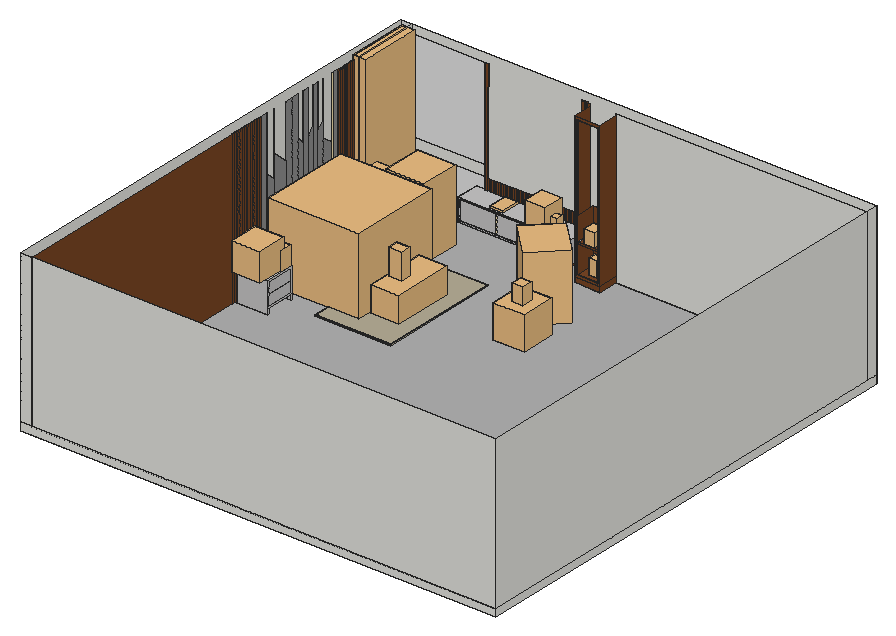
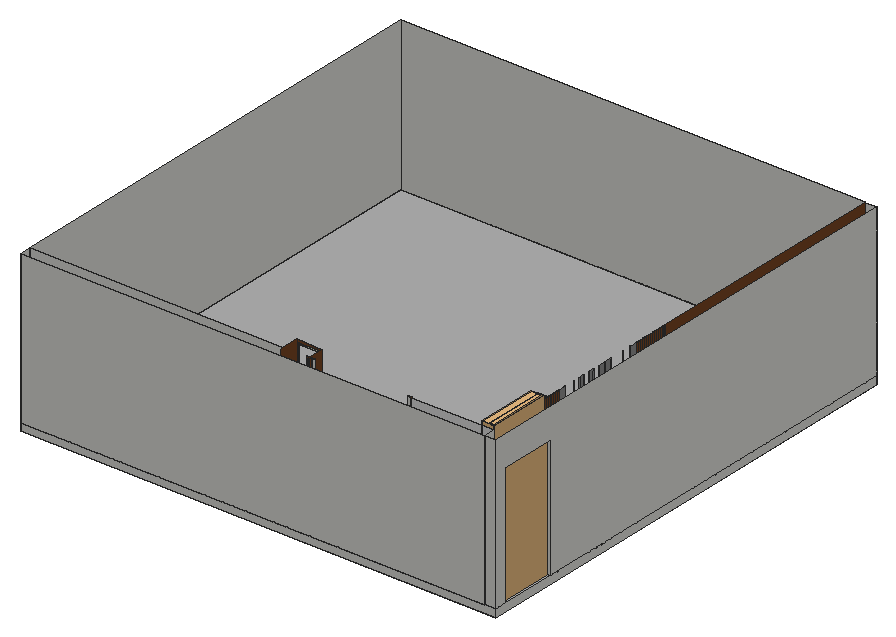
# SketchUp Ruby script. Lengths in inches.
U = 1.inch
M = Sketchup.active_model
def pt(a) = Geom::Point3d.new(a.map { |v| v * U })
def face(e, loops, mat)
  f = e.add_face(loops[0].map { |a| pt(a) })
  loops[1..].each { |l| e.add_face(l.map { |a| pt(a) }).erase! }
  f.material = f.back_material = mat if mat
  f
end
# faces: each face lists its corners as indices into pts; further lists are holes
def faces(e, pts, list, mat = nil) = list.each { |f| face(e, (f[0].is_a?(Array) ? f : [f]).map { |l| l.map { |i| pts[i] } }, mat) }
# xy, xz, yz: faces in a plane at the given z, y or x. An outline is a flat list of corners, or four numbers for a rectangle; further outlines are holes
def ring(l) = l.size == 4 ? [[l[0], l[1]], [l[2], l[1]], [l[2], l[3]], [l[0], l[3]]] : l.each_slice(2).to_a
def flat(e, list, mat, &to3) = list.each { |f| face(e, (f[0].is_a?(Array) ? f : [f]).map { |l| ring(l).map { |u, v| to3.(u, v) } }, mat) }
def xy(e, z, list, mat = nil) = flat(e, list, mat) { |x, y| [x, y, z] }
def xz(e, y, list, mat = nil) = flat(e, list, mat) { |x, z| [x, y, z] }
def yz(e, x, list, mat = nil) = flat(e, list, mat) { |y, z| [x, y, z] }
def lines(e, pts, list) = list.each { |a, b| e.add_line(pt(pts[a]), pt(pts[b])) }
# prism: a flat outline (further loops are holes) pulled along v
def prism(e, loops, v, mat = nil)
  f = face(e, loops, mat); d = Geom::Vector3d.new(v.map { |x| x * U })
  f.pushpull(f.normal.samedirection?(d) ? d.length : -d.length)
end
def box(e, o, s, mat = nil) = prism(e, [[o, [o[0] + s[0], o[1], o[2]], [o[0] + s[0], o[1] + s[1], o[2]], [o[0], o[1] + s[1], o[2]]]], [0, 0, s[2]], mat)
def at(x, y, z, deg = 0) = Geom::Transformation.translation(pt([x, y, z])) * Geom::Transformation.rotation(ORIGIN, Z_AXIS, deg.degrees)
def axes(o, x, y, z) = Geom::Transformation.new([*x, 0, *y, 0, *z, 0, *pt(o).to_a, 1])
def part(name) = M.definitions.add(name)
# library, detail: a bought-in or finely detailed component or shape, given as its bounding box
def library(name, o, s) = part(name).tap { |d| box(d.entities, o, s) }
def detail(e, o, s) = box(e.add_group.entities, o, s)
def put(e, d, t, mat = nil) = e.add_instance(d, t).tap { |i| i.material = mat if mat }
def group(e, t, mat = nil) = e.add_group.tap { |g| g.transformation = t; g.material = mat if mat }.entities
root = M.entities
M.materials.add("Ashlee 5_ x 8_").color = [182, 173, 150]
M.materials.add("Emissive").color = [234, 236, 196]
M.materials.add("Generic").color = [198, 197, 197]
M.materials.add("Gold 10k").color = [251, 232, 180]
M.materials.add("Tiles Simple J01 100cm").color = [178, 178, 178]
M.materials.add("[Color M01]").color = [226, 226, 226]
M.materials.add("[Color M04]").color = [142, 142, 142]
M.materials.add("[Wood Veneer 01]").color = [120, 70, 37]
c1 = library("Window 46-12",[-37.28,-2.15,0],[74.56,4.3,92.91])
c2 = library("Granville Side Chair",[-10.69,-11.14,0],[21.38,22.37,32.46])
c3 = part(" rug 5'x8'\#1")
xy(c3.entities,0,[[0,0,60,96]],"Ashlee 5_ x 8_")
xy(c3.entities,0.75,[[0.25,0.25,59.75,95.75]],"Ashlee 5_ x 8_")
xz(c3.entities,0,[[0,0,60,0.5]],"Ashlee 5_ x 8_")
xz(c3.entities,96,[[0,0,60,0.5]],"Ashlee 5_ x 8_")
yz(c3.entities,0,[[0,0,96,0.5]],"Ashlee 5_ x 8_")
yz(c3.entities,60,[[0,0,96,0.5]],"Ashlee 5_ x 8_")
p = [[59.99,0.01,0.56],[0.01,0.01,0.56],[0,0,0.5],[60,0,0.5],[0.01,95.99,0.56],[0,96,0.5],
  [59.99,95.99,0.56],[60,96,0.5],[0.03,0.03,0.625],[0.03,95.97,0.625],[59.97,0.03,0.625],[59.93,0.07,0.68],
  [0.07,0.07,0.68],[0.07,95.93,0.68],[59.93,95.93,0.68],[59.97,95.97,0.625],[0.125,0.125,0.72],[0.125,95.875,0.72],
  [59.81,0.19,0.74],[0.19,0.19,0.74],[59.875,0.125,0.72],[0.19,95.81,0.74],[59.81,95.81,0.74],[59.875,95.875,0.72],
  [0.25,0.25,0.75],[0.25,95.75,0.75],[59.75,0.25,0.75],[59.75,95.75,0.75]]
faces(c3.entities,p,[[0,1,2,3],[1,4,5,2],[6,0,3,7],[4,6,7,5],[8,9,4,1],[10,8,1,0],[11,12,8,10],[12,13,9,8],
  [14,11,10,15],[15,10,0,6],[13,14,15,9],[9,15,6,4],[16,17,13,12],[18,19,16,20],[20,16,12,11],[19,21,17,16],
  [22,18,20,23],[23,20,11,14],[24,25,21,19],[26,24,19,18],[27,26,18,22],[21,22,23,17],[25,27,22,21],[17,23,14,13]],"Ashlee 5_ x 8_")
c4 = library("Granville Bridge Armchair",[-12.42,-11.18,0],[24.84,22.36,32.46])
c5 = library("Bed 003",[-38.05,-87.1,0],[75.86,87.1,55.12])
c6 = library("Negro Coffee Table",[-11.41,-11.39,0.01],[22.79,22.78,16.72])
c7 = library("Eva Bench",[-23.95,-11.14,0],[47.9,22.28,20.23])
c8 = library("Curtains 005",[-39.6,-1.86,0],[79.2,3.72,117.07])
c9 = library("Curtains 47-24",[-33.71,-5.15,0],[67.39,10.25,93.3])
c10 = library("Milk Jug 92-23",[-3.1,-3.1,0],[6.18,6.2,11.88])
c11 = library("Vase 20-10",[-4.83,-4.83,0],[9.66,9.66,14.63])
c12 = library("Vase Roses 63-11",[-11.16,-11.66,0.01],[22.4,23.28,22.51])
c13 = library("Vase 003",[-5.32,-3.71,0],[10.44,8.14,20.48])
c14 = library("Calla Lilies 63-10",[-4.34,-4.49,0],[8.67,8.83,13.09])
c15 = library("Vase 005",[-3.71,-4.3,0.02],[8.35,9.45,10.71])
c16 = library("Book 298 011 003",[-5.11,-7.51,-0.03],[10.21,15.02,1.37])
c17 = library("Vase 012",[-2.85,-2.85,0],[5.7,5.7,9.98])
c18 = library("Vase Calla Lilies 21-24",[-7.55,-8.25,0],[16.06,16.68,17.86])
xy(root,-6,[[0,0,376.875,376.875]])
xy(root,0,[[0,0,0,322.76,9,322.76,9,321.04,8.75,321.04,8.75,318.98,9,318.98,9,317.73,8.75,317.73,8.75,316.79,9,316.79,9,315.55,8.75,315.55,8.75,314.73,9,314.73,9,313.48,8.75,313.48,8.75,312.66,9,312.66,9,311.42,9.0625,311.42,9.0625,310.66,9,310.66,9,309.42,9.0625,309.42,9.0625,308.48,9,308.48,9,307.23,9.0625,307.23,9.0625,306.48,9,306.48,9,305.23,9.0625,305.23,9.0625,304.35,9,304.35,9,303.11,8.625,303.11,8.625,298.11,9.125,298.11,9.125,297.48,9,297.48,9,288.56,8.9375,288.56,8.9375,288.31,9,288.31,9,283.12,8.9375,283.12,8.9375,282.87,9,282.87,9,279.06,8.9375,279.06,8.9375,278.81,9,278.81,9,274.12,8.9375,274.12,8.9375,273.87,9,273.87,9,269.18,8.9375,269.18,8.9375,268.93,9,268.93,9,263.87,8.9375,263.87,8.9375,263.62,9,263.62,9,258.18,8.9375,258.18,8.9375,257.93,9,257.93,9,251.81,8.9375,251.81,8.9375,251.56,9,251.56,9,240.43,8.9375,240.43,8.9375,240.18,9,240.18,9,233,9.125,233,9.125,232.43,8.625,232.43,8.625,227.43,9,227.43,9,226.19,8.75,226.19,8.75,225.48,9,225.48,9,224.24,8.75,224.24,8.75,223.52,9,223.52,9,222.28,8.75,222.28,8.75,221.57,9,221.57,9,220.33,8.75,220.33,8.75,219.62,9,219.62,9,218.37,8.75,218.37,8.75,217.66,9,217.66,9,216.42,8.75,216.42,8.75,215.71,9,215.71,9,214.46,8.75,214.46,8.75,213.75,9,213.75,9,212.51,8.75,212.51,8.75,211.8,9,211.8,9,210.56,8.75,210.56,8.75,209.84,9,209.84,9,208.6,8.75,208.6,8.75,207.89,9,207.89,9,206.65,8.75,206.65,8.75,205.93,9,205.93,9,204.69,8.75,204.69,8.75,203.98,9,203.98,9,202.74,8.75,202.74,8.75,202.03,9,202.03,9,200.78,8.75,200.78,8.75,200.07,9,200.07,9,198.83,8.75,198.83,8.75,198.12,9,198.12,9,0],[10.6875,201.5,10.6875,225.5,34.6875,225.5,34.6875,224.5,12.6875,224.5,12.6875,202.5,34.6875,202.5,34.6875,201.5],[10.6875,305.5,10.6875,329.5,34.6875,329.5,34.6875,328.5,12.6875,328.5,12.6875,306.5,34.6875,306.5,34.6875,305.5],[157.58,351.875,177.89,351.875,177.89,367.875,376.875,367.875,376.875,376.875,9,376.875,9,367.875,155.16,367.875,155.16,367.25,157.58,367.25],[0,367.875,9,376.875]])
xy(root,0,[[[9,0,376.875,0,376.875,367.875,177.89,367.875,177.89,351.875,157.58,351.875,157.58,367.25,155.16,367.25,155.16,367.875,0,367.875,0,322.76,9,322.76,9,321.04,8.75,321.04,8.75,318.98,9,318.98,9,317.73,8.75,317.73,8.75,316.79,9,316.79,9,315.55,8.75,315.55,8.75,314.73,9,314.73,9,313.48,8.75,313.48,8.75,312.66,9,312.66,9,311.42,9.0625,311.42,9.0625,310.66,9,310.66,9,309.42,9.0625,309.42,9.0625,308.48,9,308.48,9,307.23,9.0625,307.23,9.0625,306.48,9,306.48,9,305.23,9.0625,305.23,9.0625,304.35,9,304.35,9,303.11,8.625,303.11,8.625,298.11,9.125,298.11,9.125,297.48,9,297.48,9,288.56,8.9375,288.56,8.9375,288.31,9,288.31,9,283.12,8.9375,283.12,8.9375,282.87,9,282.87,9,279.06,8.9375,279.06,8.9375,278.81,9,278.81,9,274.12,8.9375,274.12,8.9375,273.87,9,273.87,9,269.18,8.9375,269.18,8.9375,268.93,9,268.93,9,263.87,8.9375,263.87,8.9375,263.62,9,263.62,9,258.18,8.9375,258.18,8.9375,257.93,9,257.93,9,251.81,8.9375,251.81,8.9375,251.56,9,251.56,9,240.43,8.9375,240.43,8.9375,240.18,9,240.18,9,233,9.125,233,9.125,232.43,8.625,232.43,8.625,227.43,9,227.43,9,226.19,8.75,226.19,8.75,225.48,9,225.48,9,224.24,8.75,224.24,8.75,223.52,9,223.52,9,222.28,8.75,222.28,8.75,221.57,9,221.57,9,220.33,8.75,220.33,8.75,219.62,9,219.62,9,218.37,8.75,218.37,8.75,217.66,9,217.66,9,216.42,8.75,216.42,8.75,215.71,9,215.71,9,214.46,8.75,214.46,8.75,213.75,9,213.75,9,212.51,8.75,212.51,8.75,211.8,9,211.8,9,210.56,8.75,210.56,8.75,209.84,9,209.84,9,208.6,8.75,208.6,8.75,207.89,9,207.89,9,206.65,8.75,206.65,8.75,205.93,9,205.93,9,204.69,8.75,204.69,8.75,203.98,9,203.98,9,202.74,8.75,202.74,8.75,202.03,9,202.03,9,200.78,8.75,200.78,8.75,200.07,9,200.07,9,198.83,8.75,198.83,8.75,198.12,9,198.12],[10.6875,201.5,10.6875,225.5,34.6875,225.5,34.6875,224.5,12.6875,224.5,12.6875,202.5,34.6875,202.5,34.6875,201.5],[10.6875,305.5,10.6875,329.5,34.6875,329.5,34.6875,328.5,12.6875,328.5,12.6875,306.5,34.6875,306.5,34.6875,305.5]]],"Tiles Simple J01 100cm")
xy(root,4,[[12.6875,202.5,34.6875,224.5],[12.6875,306.5,34.6875,328.5]])
xy(root,5.63,[[159.21,351.875,176.26,352.5625]],"[Wood Veneer 01]")
xy(root,6,[[159.58,352.5625,175.89,367.875]],"[Wood Veneer 01]")
xy(root,12,[[155.16,367.25,155.75,367.875]])
xy(root,12,[[67.16,349.875,155.75,366.875]],"Generic")
xy(root,12.25,[[67.16,366.875,67.16,367.875,155.16,367.875,155.16,367.25,155.75,367.25,155.75,366.875]],"Emissive")
xy(root,24,[[10.6875,201.5,34.6875,225.5],[10.6875,305.5,34.6875,329.5]],"Generic")
xy(root,27.59,[[159.58,352.5625,175.89,366.875]],"[Wood Veneer 01]")
xy(root,27.84,[[159.58,366.875,175.89,367.875]],"Emissive")
xy(root,28.99,[[159.58,352.5625,175.89,367.875]],"[Wood Veneer 01]")
xy(root,30,[[74.65,367.25,76.95,367.875],[78.89,367.25,81.19,367.875],[83.125,367.25,85.43,367.875],[87.36,367.25,89.67,367.875],[91.6,367.25,93.9,367.875],
  [95.84,367.25,98.14,367.875],[100.07,367.25,102.38,367.875],[104.3125,367.25,106.62,367.875],[108.55,367.25,110.85,367.875],[112.79,367.25,115.09,367.875],
  [117.02,367.25,119.33,367.875],[121.26,367.25,123.57,367.875],[125.5,367.25,127.8,367.875],[129.74,367.25,132.04,367.875],[133.97,367.25,136.28,367.875],
  [138.21,367.25,140.52,367.875],[142.45,367.25,144.75,367.875],[146.6875,367.25,148.99,367.875],[150.92,367.25,153.23,367.875],[155.16,367.25,155.75,367.875]])
xy(root,30,[[67.16,349.875,155.75,349.875,155.75,367.25,155.16,367.25,155.16,367.875,153.23,367.875,153.23,367.25,150.92,367.25,150.92,367.875,148.99,367.875,148.99,367.25,146.6875,367.25,146.6875,367.875,144.75,367.875,144.75,367.25,142.45,367.25,142.45,367.875,140.52,367.875,140.52,367.25,138.21,367.25,138.21,367.875,136.28,367.875,136.28,367.25,133.97,367.25,133.97,367.875,132.04,367.875,132.04,367.25,129.74,367.25,129.74,367.875,127.8,367.875,127.8,367.25,125.5,367.25,125.5,367.875,123.57,367.875,123.57,367.25,121.26,367.25,121.26,367.875,119.33,367.875,119.33,367.25,117.02,367.25,117.02,367.875,115.09,367.875,115.09,367.25,112.79,367.25,112.79,367.875,110.85,367.875,110.85,367.25,108.55,367.25,108.55,367.875,106.62,367.875,106.62,367.25,104.3125,367.25,104.3125,367.875,102.38,367.875,102.38,367.25,100.07,367.25,100.07,367.875,98.14,367.875,98.14,367.25,95.84,367.25,95.84,367.875,93.9,367.875,93.9,367.25,91.6,367.25,91.6,367.875,89.67,367.875,89.67,367.25,87.36,367.25,87.36,367.875,85.43,367.875,85.43,367.25,83.125,367.25,83.125,367.875,81.19,367.875,81.19,367.25,78.89,367.25,78.89,367.875,76.95,367.875,76.95,367.25,74.65,367.25,74.65,367.875,67.16,367.875]],"Generic")
xz(root,0,[[0,-6,376.875,0],[0,0,9,120],[9,0,376.875,120.125]])
xz(root,198.12,[[8.75,0,9,120]],"[Wood Veneer 01]")
xz(root,198.83,[[8.75,0,9,120]],"[Wood Veneer 01]")
xz(root,200.07,[[8.75,0,9,120]],"[Wood Veneer 01]")
xz(root,200.78,[[8.75,0,9,120]],"[Wood Veneer 01]")
xz(root,201.5,[[10.6875,0,34.6875,24]],"Generic")
xz(root,202.03,[[8.75,0,9,120]],"[Wood Veneer 01]")
xz(root,202.5,[[12.6875,0,34.6875,4]],"Generic")
xz(root,202.74,[[8.75,0,9,120]],"[Wood Veneer 01]")
xz(root,203.98,[[8.75,0,9,120]],"[Wood Veneer 01]")
xz(root,204.69,[[8.75,0,9,120]],"[Wood Veneer 01]")
xz(root,205.93,[[8.75,0,9,120]],"[Wood Veneer 01]")
xz(root,206.65,[[8.75,0,9,120]],"[Wood Veneer 01]")
xz(root,207.89,[[8.75,0,9,120]],"[Wood Veneer 01]")
xz(root,208.6,[[8.75,0,9,120]],"[Wood Veneer 01]")
xz(root,209.84,[[8.75,0,9,120]],"[Wood Veneer 01]")
xz(root,210.56,[[8.75,0,9,120]],"[Wood Veneer 01]")
xz(root,211.8,[[8.75,0,9,120]],"[Wood Veneer 01]")
xz(root,212.51,[[8.75,0,9,120]],"[Wood Veneer 01]")
xz(root,213.75,[[8.75,0,9,120]],"[Wood Veneer 01]")
xz(root,214.46,[[8.75,0,9,120]],"[Wood Veneer 01]")
xz(root,215.71,[[8.75,0,9,120]],"[Wood Veneer 01]")
xz(root,216.42,[[8.75,0,9,120]],"[Wood Veneer 01]")
xz(root,217.66,[[8.75,0,9,120]],"[Wood Veneer 01]")
xz(root,218.37,[[8.75,0,9,120]],"[Wood Veneer 01]")
xz(root,219.62,[[8.75,0,9,120]],"[Wood Veneer 01]")
xz(root,220.33,[[8.75,0,9,120]],"[Wood Veneer 01]")
xz(root,221.57,[[8.75,0,9,120]],"[Wood Veneer 01]")
xz(root,222.28,[[8.75,0,9,120]],"[Wood Veneer 01]")
xz(root,223.52,[[8.75,0,9,120]],"[Wood Veneer 01]")
xz(root,224.24,[[8.75,0,9,120]],"[Wood Veneer 01]")
xz(root,224.5,[[12.6875,0,34.6875,4]],"Generic")
xz(root,225.48,[[8.75,0,9,120]],"[Wood Veneer 01]")
xz(root,225.5,[[10.6875,0,34.6875,24]])
xz(root,226.19,[[8.75,0,9,120]],"[Wood Veneer 01]")
xz(root,227.43,[[8.625,0,9,120]],"Emissive")
xz(root,232.43,[[8.625,0,9.125,120]],"Gold 10k")
xz(root,233,[[9,0,9,76.84,8.9375,76.84,8.9375,77.53,9,77.53,9,83.85,8.9375,83.85,8.9375,84.85,9,84.85,9,120,9.125,120,9.125,0]],"Gold 10k")
xz(root,240.18,[[8.9375,0,9,70.25]])
xz(root,240.43,[[8.9375,0,9,87.71]],"[Color M04]")
xz(root,251.56,[[8.9375,0,9,77.93]])
xz(root,251.81,[[8.9375,0,9,120]],"[Color M04]")
xz(root,257.93,[[8.9375,0,9,120]])
xz(root,258.18,[[8.9375,0,9,120]],"[Color M04]")
xz(root,263.62,[[8.9375,0,9,120]],"[Color M04]")
xz(root,263.87,[[8.9375,0,9,89.29]],"[Color M04]")
xz(root,268.93,[[8.9375,0,9,83.18]],"[Color M04]")
xz(root,269.18,[[8.9375,0,9,120]],"[Color M04]")
xz(root,273.87,[[8.9375,0,9,120]],"[Color M04]")
xz(root,274.12,[[8.9375,0,9,86.125]],"[Color M04]")
xz(root,278.81,[[8.9375,0,9,90.68]],"[Color M04]")
xz(root,279.06,[[8.9375,0,9,120]],"[Color M04]")
xz(root,282.87,[[8.9375,0,9,120]],"[Color M04]")
xz(root,283.12,[[8.9375,0,9,86.5]],"[Color M04]")
xz(root,288.31,[[8.9375,0,9,89.6]],"[Color M04]")
xz(root,288.56,[[8.9375,0,9,78.14]])
xz(root,297.48,[[9,0,9.125,0,9.125,120,9,120,9,106.14,8.9375,106.14,8.9375,105.77,9,105.77,9,71.82,8.9375,71.82,8.9375,71.32,9,71.32]],"Gold 10k")
xz(root,298.11,[[8.625,0,9.125,120]],"Gold 10k")
xz(root,303.11,[[8.625,0,9,120]],"Emissive")
xz(root,304.35,[[9,0,9.0625,120]],"[Wood Veneer 01]")
xz(root,305.23,[[9,0,9.0625,120]],"[Wood Veneer 01]")
xz(root,305.5,[[10.6875,0,34.6875,24]],"Generic")
xz(root,306.48,[[9,0,9.0625,120]],"[Wood Veneer 01]")
xz(root,306.5,[[12.6875,0,34.6875,4]],"Generic")
xz(root,307.23,[[9,0,9.0625,120]],"[Wood Veneer 01]")
xz(root,308.48,[[9,0,9.0625,120]],"[Wood Veneer 01]")
xz(root,309.42,[[9,0,9.0625,120]],"[Wood Veneer 01]")
xz(root,310.66,[[9,0,9.0625,120]],"[Wood Veneer 01]")
xz(root,311.42,[[9,0,9.0625,120]],"[Wood Veneer 01]")
xz(root,312.66,[[8.75,0,9,120]],"[Wood Veneer 01]")
xz(root,313.48,[[8.75,0,9,120]],"[Wood Veneer 01]")
xz(root,314.73,[[8.75,0,9,120]],"[Wood Veneer 01]")
xz(root,315.55,[[8.75,0,9,120]],"[Wood Veneer 01]")
xz(root,316.79,[[8.75,0,9,120]],"[Wood Veneer 01]")
xz(root,317.73,[[8.75,0,9,120]],"[Wood Veneer 01]")
xz(root,318.98,[[8.75,0,9,120]],"[Wood Veneer 01]")
xz(root,321.04,[[8.75,0,9,120]],"[Wood Veneer 01]")
xz(root,322.76,[[0,0,9,96]])
xz(root,328.5,[[12.6875,0,34.6875,4]],"Generic")
xz(root,329.5,[[10.6875,0,34.6875,24]],"Generic")
xz(root,349.875,[[[67.16,12,155.75,30],[68.16,13,154.75,29]],[68.5625,13.4,97.16,28.6],[97.56,13.4,125.75,28.6],[126.15,13.4,154.35,28.6]],"Generic")
xz(root,349.875,[[[68.16,13,154.75,29],[68.5625,13.4,154.35,28.6]],[97.16,13.4,97.56,28.6],[125.75,13.4,126.15,28.6]],"Gold 10k")
xz(root,351.875,[[157.58,0,177.89,4],[[157.58,4,177.89,118],[159.21,5.63,176.26,116.37]]],"[Wood Veneer 01]")
xz(root,352.5625,[[[159.21,5.63,176.26,116.37],[159.58,6,175.89,116]]],"Emissive")
xz(root,352.5625,[[159.58,27.59,175.89,28.99]],"[Wood Veneer 01]")
xz(root,366.875,[[67.16,12,155.75,12.25],[159.58,27.59,175.89,27.84]],"Emissive")
xz(root,367.25,[[155.16,12,155.75,12.25]],"Emissive")
xz(root,367.25,[[155.16,0,157.58,0,157.58,120,155.16,120,155.16,30,155.75,30,155.75,12,155.16,12],[74.65,30,76.95,30,76.95,38.375,76.01,38.375,76.01,103.625,76.95,103.625,76.95,120,74.65,120],[78.89,30,81.19,38.625],[83.125,30,85.43,38.625],[87.36,30,89.67,38.625],
  [91.6,30,93.9,38.625],[95.84,30,98.14,38.625],[100.07,30,102.38,38.625],[104.3125,30,106.62,38.625],[108.55,30,110.85,38.625],
  [112.79,30,115.09,38.625],[117.02,30,119.33,38.625],[121.26,30,123.57,38.625],[125.5,30,127.8,38.625],[129.74,30,132.04,38.625],
  [133.97,30,136.28,38.625],[138.21,30,140.52,38.625],[142.45,30,144.75,38.625],[146.6875,30,148.99,38.625],[150.92,30,153.23,30,153.23,120,150.92,120,150.92,103.625,151.83,103.625,151.83,38.375,150.92,38.375]],"[Wood Veneer 01]")
xz(root,367.875,[[0,0,9,96],[177.89,0,376.875,120],[155.16,12,155.75,30],[67.16,12.25,74.65,30],[74.65,12.25,76.95,30],
  [76.95,12.25,78.89,30],[78.89,12.25,81.19,30],[81.19,12.25,83.125,30],[83.125,12.25,85.43,30],[85.43,12.25,87.36,30],
  [87.36,12.25,89.67,30],[89.67,12.25,91.6,30],[91.6,12.25,93.9,30],[93.9,12.25,95.84,30],[95.84,12.25,98.14,30],
  [98.14,12.25,100.07,30],[100.07,12.25,102.38,30],[102.38,12.25,104.3125,30],[104.3125,12.25,106.62,30],[106.62,12.25,108.55,30],
  [108.55,12.25,110.85,30],[110.85,12.25,112.79,30],[112.79,12.25,115.09,30],[115.09,12.25,117.02,30],[117.02,12.25,119.33,30],
  [119.33,12.25,121.26,30],[121.26,12.25,123.57,30],[123.57,12.25,125.5,30],[125.5,12.25,127.8,30],[127.8,12.25,129.74,30],
  [129.74,12.25,132.04,30],[132.04,12.25,133.97,30],[133.97,12.25,136.28,30],[136.28,12.25,138.21,30],[138.21,12.25,140.52,30],
  [140.52,12.25,142.45,30],[142.45,12.25,144.75,30],[144.75,12.25,146.6875,30],[146.6875,12.25,148.99,30],[148.99,12.25,150.92,30],
  [150.92,12.25,153.23,30],[153.23,12.25,155.16,30],[159.58,27.84,175.89,28.99],[74.65,30,74.65,120,76.95,120,76.95,103.625,76.01,103.625,76.01,38.375,76.95,38.375,76.95,30],[150.92,30,153.23,30,153.23,120,150.92,120,150.92,103.625,151.83,103.625,151.83,38.375,150.92,38.375]])
xz(root,367.875,[[[9,0,74.65,0,74.65,12.25,67.16,12.25,67.16,30,74.65,30,74.65,120,9,120],[14.5,38.375,73.93,47.375]]],"[Color M01]")
xz(root,367.875,[[74.65,0,76.95,12.25],[76.95,0,78.89,12.25],[78.89,0,81.19,12.25],[81.19,0,83.125,12.25],[83.125,0,85.43,12.25],
  [85.43,0,87.36,12.25],[87.36,0,89.67,12.25],[89.67,0,91.6,12.25],[91.6,0,93.9,12.25],[93.9,0,95.84,12.25],
  [95.84,0,98.14,12.25],[98.14,0,100.07,12.25],[100.07,0,102.38,12.25],[102.38,0,104.3125,12.25],[104.3125,0,106.62,12.25],
  [106.62,0,108.55,12.25],[108.55,0,110.85,12.25],[110.85,0,112.79,12.25],[112.79,0,115.09,12.25],[115.09,0,117.02,12.25],
  [117.02,0,119.33,12.25],[119.33,0,121.26,12.25],[121.26,0,123.57,12.25],[123.57,0,125.5,12.25],[125.5,0,127.8,12.25],
  [127.8,0,129.74,12.25],[129.74,0,132.04,12.25],[132.04,0,133.97,12.25],[133.97,0,136.28,12.25],[136.28,0,138.21,12.25],
  [138.21,0,140.52,12.25],[140.52,0,142.45,12.25],[142.45,0,144.75,12.25],[144.75,0,146.6875,12.25],[146.6875,0,148.99,12.25],
  [148.99,0,150.92,12.25],[150.92,0,153.23,12.25],[153.23,0,155.16,12.25],[159.58,6,175.89,27.84],[159.58,28.99,175.89,47.84],
  [76.95,30,78.89,38.375],[81.19,30,83.125,38.375],[85.43,30,87.36,38.375],[89.67,30,91.6,38.375],[93.9,30,95.84,38.375],
  [98.14,30,100.07,38.375],[102.38,30,104.3125,38.375],[106.62,30,108.55,38.375],[110.85,30,112.79,38.375],[115.09,30,117.02,38.375],
  [119.33,30,121.26,38.375],[123.57,30,125.5,38.375],[127.8,30,129.74,38.375],[132.04,30,133.97,38.375],[136.28,30,138.21,38.375],
  [140.52,30,142.45,38.375],[144.75,30,146.6875,38.375],[148.99,30,150.92,38.375],[153.23,30,155.16,120]],"[Wood Veneer 01]")
xz(root,376.875,[[0,-6,376.875,0],[0,0,9,120],[9,0,376.875,120]])
yz(root,0,[[0,-6,376.875,0],[0,0,0,120,376.875,120,376.875,0,367.875,0,367.875,96,322.76,96,322.76,0]])
yz(root,8.625,[[227.43,0,232.43,120],[298.11,0,303.11,120]],"[Color M04]")
yz(root,8.75,[[198.12,0,198.83,120],[200.07,0,200.78,120],[202.03,0,202.74,120],[203.98,0,204.69,120],[205.93,0,206.65,120],
  [207.89,0,208.6,120],[209.84,0,210.56,120],[211.8,0,212.51,120],[213.75,0,214.46,120],[215.71,0,216.42,120],
  [217.66,0,218.37,120],[219.62,0,220.33,120],[221.57,0,222.28,120],[223.52,0,224.24,120],[225.48,0,226.19,120],
  [312.66,0,313.48,120],[314.73,0,315.55,120],[316.79,0,317.73,120],[318.98,0,319.8,120],[319.8,0,321.04,120]],"[Wood Veneer 01]")
yz(root,8.9375,[[240.18,0,240.43,120],[251.56,0,251.81,120],[257.93,0,258.18,120],[263.62,0,263.87,120],[268.93,0,269.18,120],
  [273.87,0,274.12,120],[278.81,0,279.06,120],[282.87,0,283.12,120],[288.31,0,288.56,120]],"[Color M04]")
yz(root,9,[[367.875,0,376.875,120]])
yz(root,9,[[233,0,240.18,0,240.18,70.25,233,76.84],[240.43,0,251.56,0,251.56,77.93,240.43,87.71],[251.81,0,257.93,120],[258.18,0,263.62,120],[263.87,0,268.93,0,268.93,83.18,263.87,89.29],
  [269.18,0,273.87,120],[274.12,0,278.81,0,278.81,90.68,274.12,86.125],[279.06,0,282.87,120],[283.12,0,288.31,0,288.31,89.6,283.12,86.5],[288.56,0,297.48,0,297.48,71.32,288.56,78.14]],"[Color M04]")
yz(root,9,[[0,0,198.12,120],[198.83,0,200.07,120],[200.78,0,202.03,120],[202.74,0,203.98,120],[204.69,0,205.93,120],
  [206.65,0,207.89,120],[208.6,0,209.84,120],[210.56,0,211.8,120],[212.51,0,213.75,120],[214.46,0,215.71,120],
  [216.42,0,217.66,120],[218.37,0,219.62,120],[220.33,0,221.57,120],[222.28,0,223.52,120],[224.24,0,225.48,120],
  [226.19,0,227.43,120],[303.11,0,304.35,120],[305.23,0,306.48,120],[307.23,0,308.48,120],[309.42,0,310.66,120],
  [311.42,0,312.66,120],[313.48,0,314.73,120],[315.55,0,316.79,120],[317.73,0,318.98,120],[321.04,0,322.76,0,322.76,96,367.875,96,367.875,120,321.04,120]],"[Wood Veneer 01]")
yz(root,9.0625,[[304.35,0,305.23,120],[306.48,0,307.23,120],[308.48,0,309.42,120],[310.66,0,311.42,120]],"[Wood Veneer 01]")
yz(root,9.125,[[232.43,0,233,120],[297.48,0,298.11,120]],"Gold 10k")
yz(root,10.6875,[[201.5,0,225.5,24],[305.5,0,329.5,24]])
yz(root,12.6875,[[306.5,0,328.5,4]])
yz(root,12.6875,[[202.5,0,224.5,4]],"Generic")
yz(root,34.6875,[[201.5,0,202.5,4],[224.5,0,225.5,4],[305.5,0,306.5,4],[328.5,0,329.5,4],[[201.5,4,225.5,24],[202.5,5,224.5,23]],
  [[305.5,4,329.5,24],[306.5,5,328.5,23]],[202.9,5.4,224.1,13.6],[306.9,5.4,328.1,13.6],[202.9,14,224.1,22.6],[306.9,14,328.1,22.6]],"Generic")
yz(root,34.6875,[[[202.5,5,224.5,23],[202.9,5.4,224.1,22.6]],[[306.5,5,328.5,23],[306.9,5.4,328.1,22.6]],[202.9,13.6,224.1,14],[306.9,13.6,328.1,14]],"Gold 10k")
yz(root,67.16,[[349.875,12,349.875,30,367.875,30,367.875,12.25,366.875,12.25,366.875,12]])
yz(root,74.65,[[367.25,30,367.875,120]],"[Wood Veneer 01]")
yz(root,76.95,[[367.25,30,367.875,38.375]],"[Wood Veneer 01]")
yz(root,78.89,[[367.25,30,367.875,38.375]])
yz(root,81.19,[[367.25,30,367.875,38.375]],"[Wood Veneer 01]")
yz(root,83.125,[[367.25,30,367.875,38.375]])
yz(root,85.43,[[367.25,30,367.875,38.375]],"[Wood Veneer 01]")
yz(root,87.36,[[367.25,30,367.875,38.375]],"[Wood Veneer 01]")
yz(root,89.67,[[367.25,30,367.875,38.375]],"[Wood Veneer 01]")
yz(root,91.6,[[367.25,30,367.875,38.375]],"[Wood Veneer 01]")
yz(root,93.9,[[367.25,30,367.875,38.375]],"[Wood Veneer 01]")
yz(root,95.84,[[367.25,30,367.875,38.375]],"[Wood Veneer 01]")
yz(root,98.14,[[367.25,30,367.875,38.375]],"[Wood Veneer 01]")
yz(root,100.07,[[367.25,30,367.875,38.375]],"[Wood Veneer 01]")
yz(root,102.38,[[367.25,30,367.875,38.375]],"[Wood Veneer 01]")
yz(root,104.3125,[[367.25,30,367.875,38.375]],"[Wood Veneer 01]")
yz(root,106.62,[[367.25,30,367.875,38.375]],"[Wood Veneer 01]")
yz(root,108.55,[[367.25,30,367.875,38.375]],"[Wood Veneer 01]")
yz(root,110.85,[[367.25,30,367.875,38.375]],"[Wood Veneer 01]")
yz(root,112.79,[[367.25,30,367.875,38.375]],"[Wood Veneer 01]")
yz(root,115.09,[[367.25,30,367.875,38.375]],"[Wood Veneer 01]")
yz(root,117.02,[[367.25,30,367.875,38.375]],"[Wood Veneer 01]")
yz(root,119.33,[[367.25,30,367.875,38.375]],"[Wood Veneer 01]")
yz(root,121.26,[[367.25,30,367.875,38.375]],"[Wood Veneer 01]")
yz(root,123.57,[[367.25,30,367.875,38.375]],"[Wood Veneer 01]")
yz(root,125.5,[[367.25,30,367.875,38.375]],"[Wood Veneer 01]")
yz(root,127.8,[[367.25,30,367.875,38.375]],"[Wood Veneer 01]")
yz(root,129.74,[[367.25,30,367.875,38.375]],"[Wood Veneer 01]")
yz(root,132.04,[[367.25,30,367.875,38.375]],"[Wood Veneer 01]")
yz(root,133.97,[[367.25,30,367.875,38.375]],"[Wood Veneer 01]")
yz(root,136.28,[[367.25,30,367.875,38.375]],"[Wood Veneer 01]")
yz(root,138.21,[[367.25,30,367.875,38.375]],"[Wood Veneer 01]")
yz(root,140.52,[[367.25,30,367.875,38.375]],"[Wood Veneer 01]")
yz(root,142.45,[[367.25,30,367.875,38.375]],"[Wood Veneer 01]")
yz(root,144.75,[[367.25,30,367.875,38.375]],"[Wood Veneer 01]")
yz(root,146.6875,[[367.25,30,367.875,38.375]],"[Wood Veneer 01]")
yz(root,148.99,[[367.25,30,367.875,38.375]],"[Wood Veneer 01]")
yz(root,150.92,[[367.25,30,367.875,38.375]],"[Wood Veneer 01]")
yz(root,153.23,[[367.25,30,367.875,120]],"[Wood Veneer 01]")
yz(root,155.16,[[367.25,12,367.875,12.25]],"Emissive")
yz(root,155.16,[[367.25,0,367.875,12],[367.25,30,367.875,120]],"[Wood Veneer 01]")
yz(root,155.75,[[367.25,12,367.875,30]])
yz(root,155.75,[[349.875,12,366.875,12,366.875,12.25,367.25,12.25,367.25,30,349.875,30]],"Generic")
yz(root,157.58,[[351.875,0,367.25,4],[351.875,4,367.25,118]],"[Wood Veneer 01]")
yz(root,159.21,[[351.875,5.63,352.5625,116.37]],"[Wood Veneer 01]")
yz(root,159.58,[[352.5625,27.59,366.875,27.59,366.875,27.84,367.875,27.84,367.875,28.99,352.5625,28.99]])
yz(root,159.58,[[352.5625,6,367.875,6,367.875,27.84,366.875,27.84,366.875,27.59,352.5625,27.59],[352.5625,28.99,367.875,28.99,367.875,47.84,366.875,47.84,366.875,47.59,352.5625,47.59]],"[Wood Veneer 01]")
yz(root,175.89,[[352.5625,27.59,352.5625,28.99,367.875,28.99,367.875,27.84,366.875,27.84,366.875,27.59]])
yz(root,175.89,[[352.5625,6,352.5625,27.59,366.875,27.59,366.875,27.84,367.875,27.84,367.875,6],[352.5625,28.99,352.5625,47.59,366.875,47.59,366.875,47.84,367.875,47.84,367.875,28.99]],"[Wood Veneer 01]")
yz(root,176.26,[[351.875,5.63,352.5625,116.37]],"[Wood Veneer 01]")
yz(root,177.89,[[351.875,0,367.875,4],[351.875,4,367.875,118]],"[Wood Veneer 01]")
yz(root,376.875,[[0,-6,376.875,0],[0,0,367.875,120.125],[367.875,0,376.875,120]])
put(root,c1,axes([4.7,344.93,-0.79],[0,0.61554,0],[-1,0,0],[0,0,1.0417]))
put(root,c2,axes([55.45,327.49,0],[-1.404,0,0],[0,-1.3794,0],[0,0,1.75398]))
put(root,c3,at(58.78,218.74,0))
put(root,c4,axes([165.31,312.53,0],[0.99702,-0.99702,0],[0.96167,0.96167,0],[0,0,1.59]))
put(root,c5,axes([10.55,268.1,0],[0,0.94908,0],[-0.82665,0,0],[0,0,1.10403]))
put(root,c6,axes([175.95,277.45,0],[1.1016,0,0],[0,1.176,0],[0,0,1.572]))
put(root,c7,at(95.35,265.66,0.75,90))
put(root,c8,axes([10.86,343.56,2.93],[0,0.6,0],[-1,0,0],[0,0,1.03]))
put(root,c9,axes([13.11,343.63,4.93],[0,0.71982,0],[-0.9408,0,0],[0,0,1.26927]))
put(root,c10,at(169.53,358.46,7.03))
put(root,c11,at(29.04,220.63,24))
put(root,c12,at(21.74,207.72,24))
put(root,c12,at(25.87,318.74,24))
put(root,c13,at(95.92,255.1,25.04))
put(root,c14,at(175.59,277.09,26.07))
put(root,c15,at(167.54,357.76,28.99))
put(root,c16,at(96.29,358.625,30))
put(root,c17,at(140.58,355.03,30))
put(root,c18,at(129.24,355.83,30))
